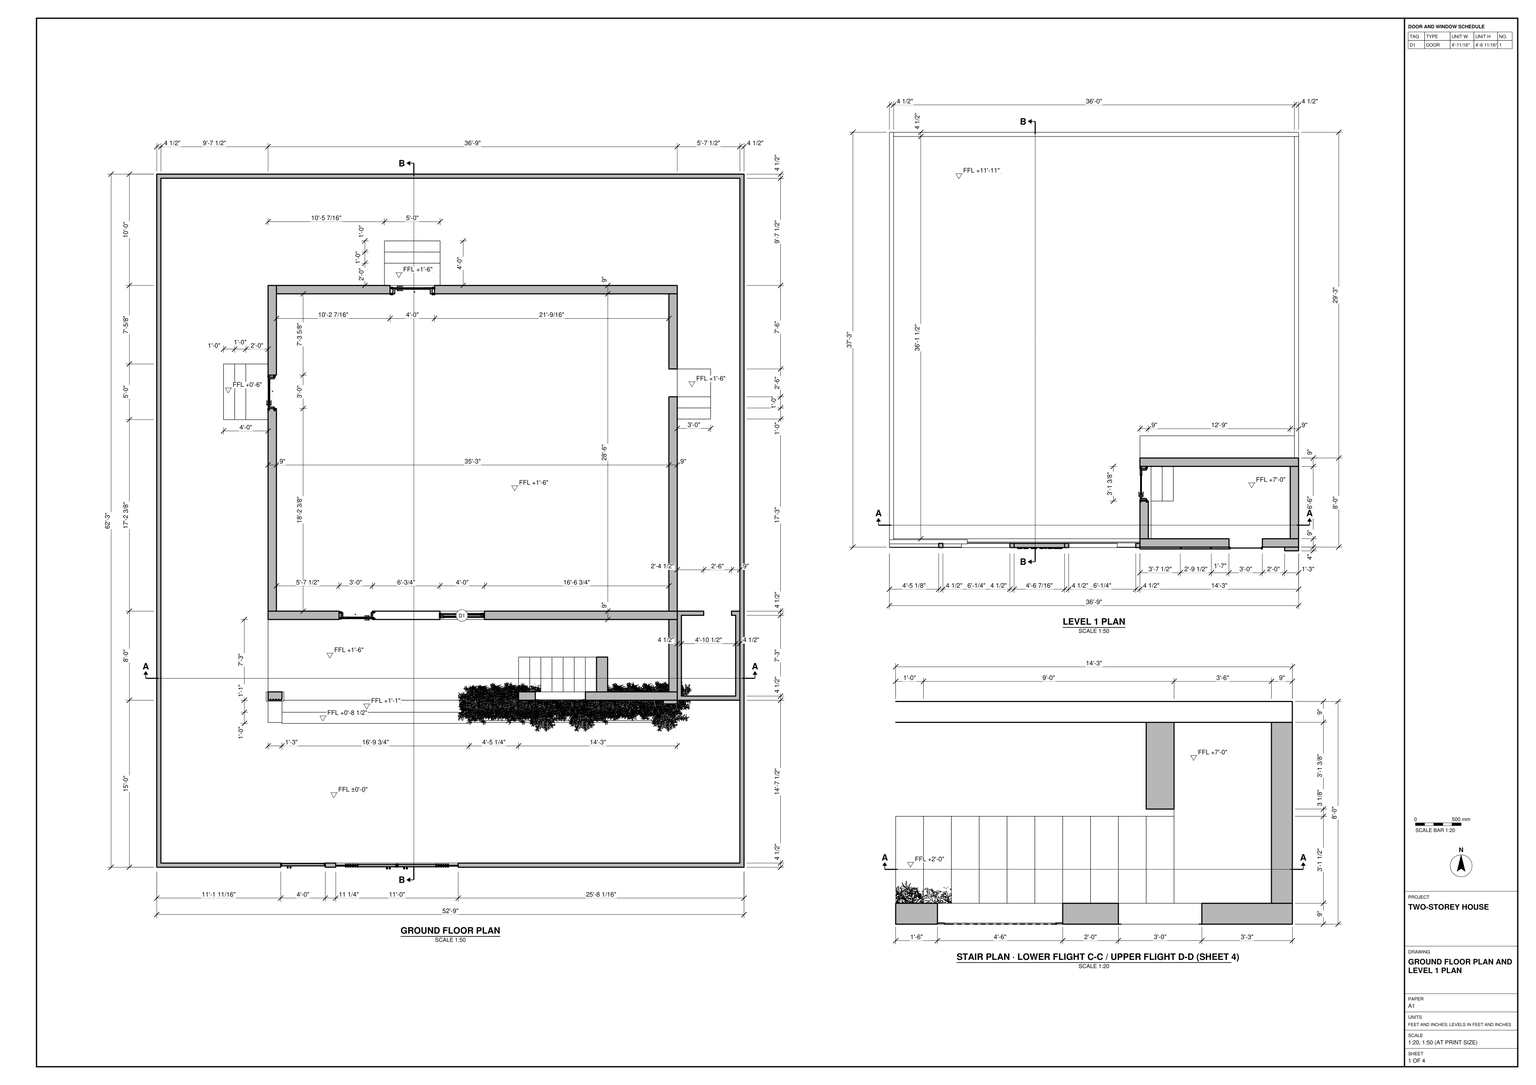
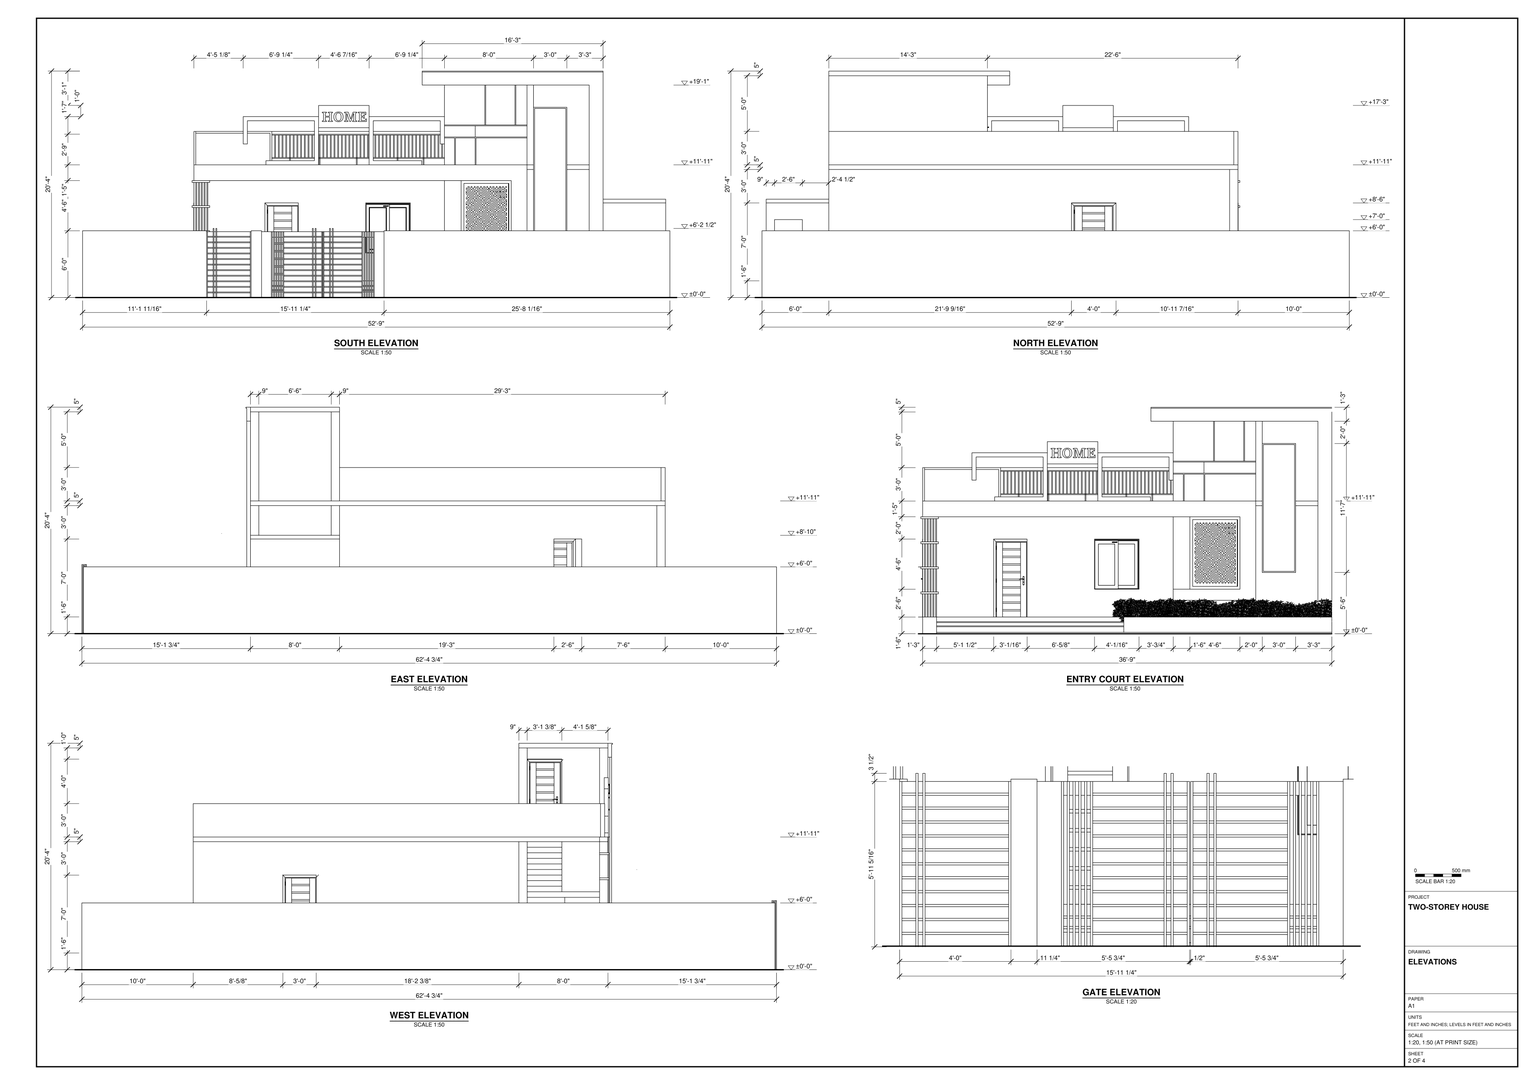
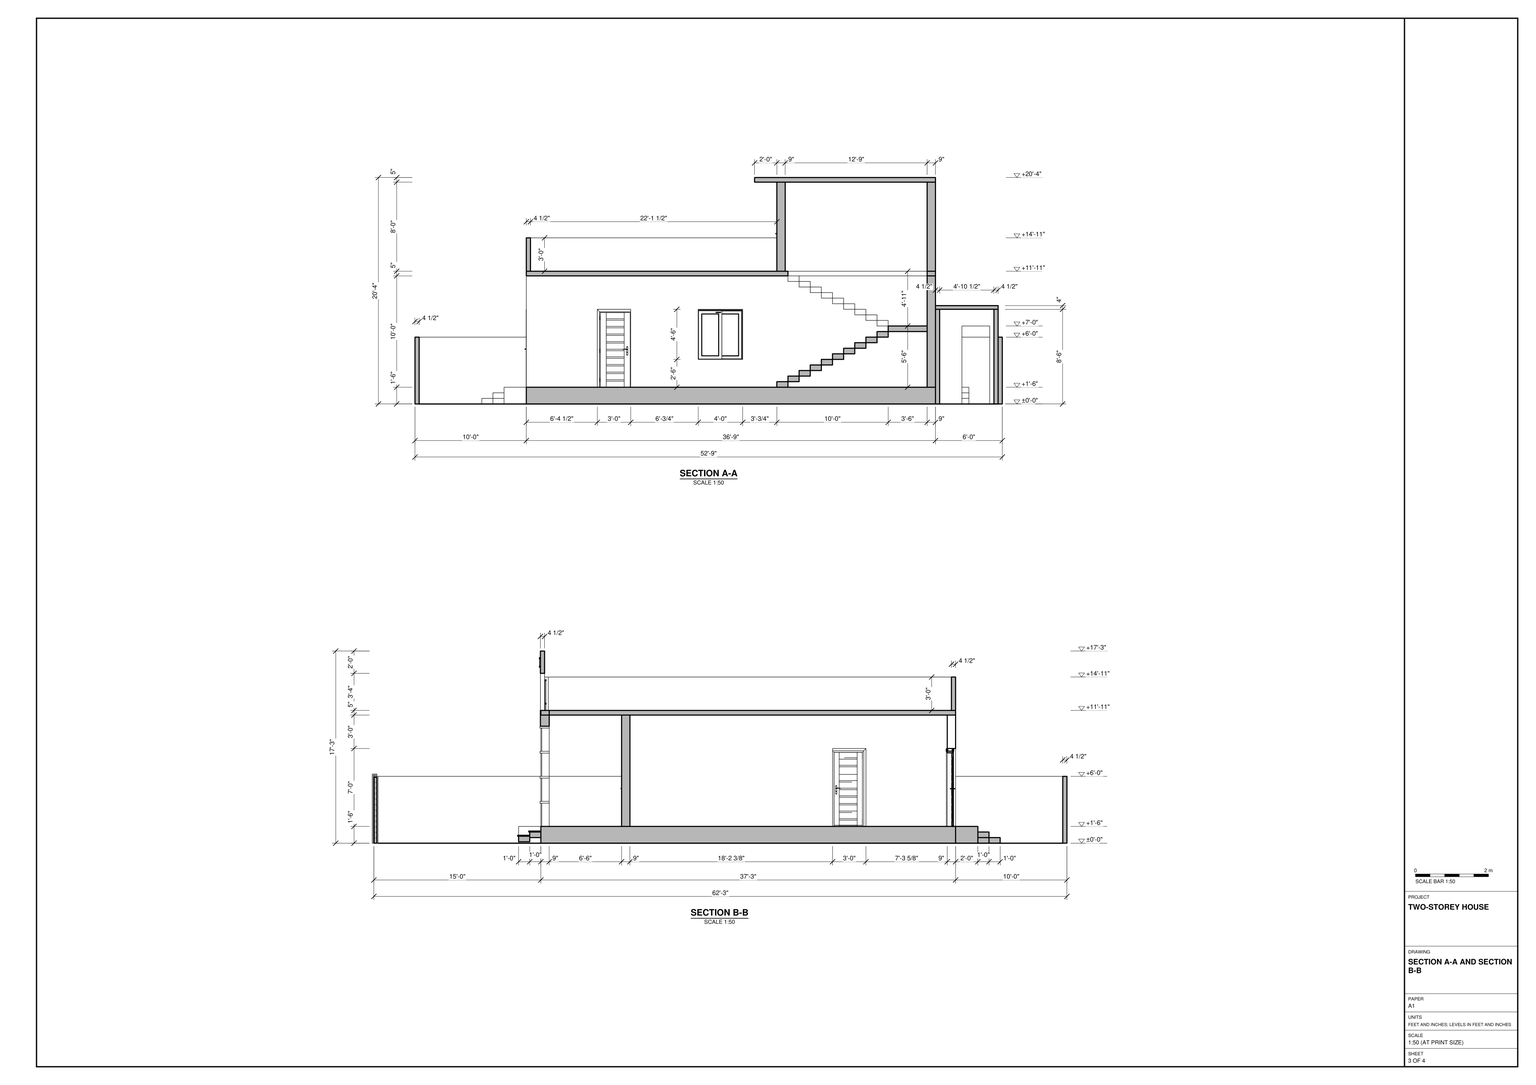
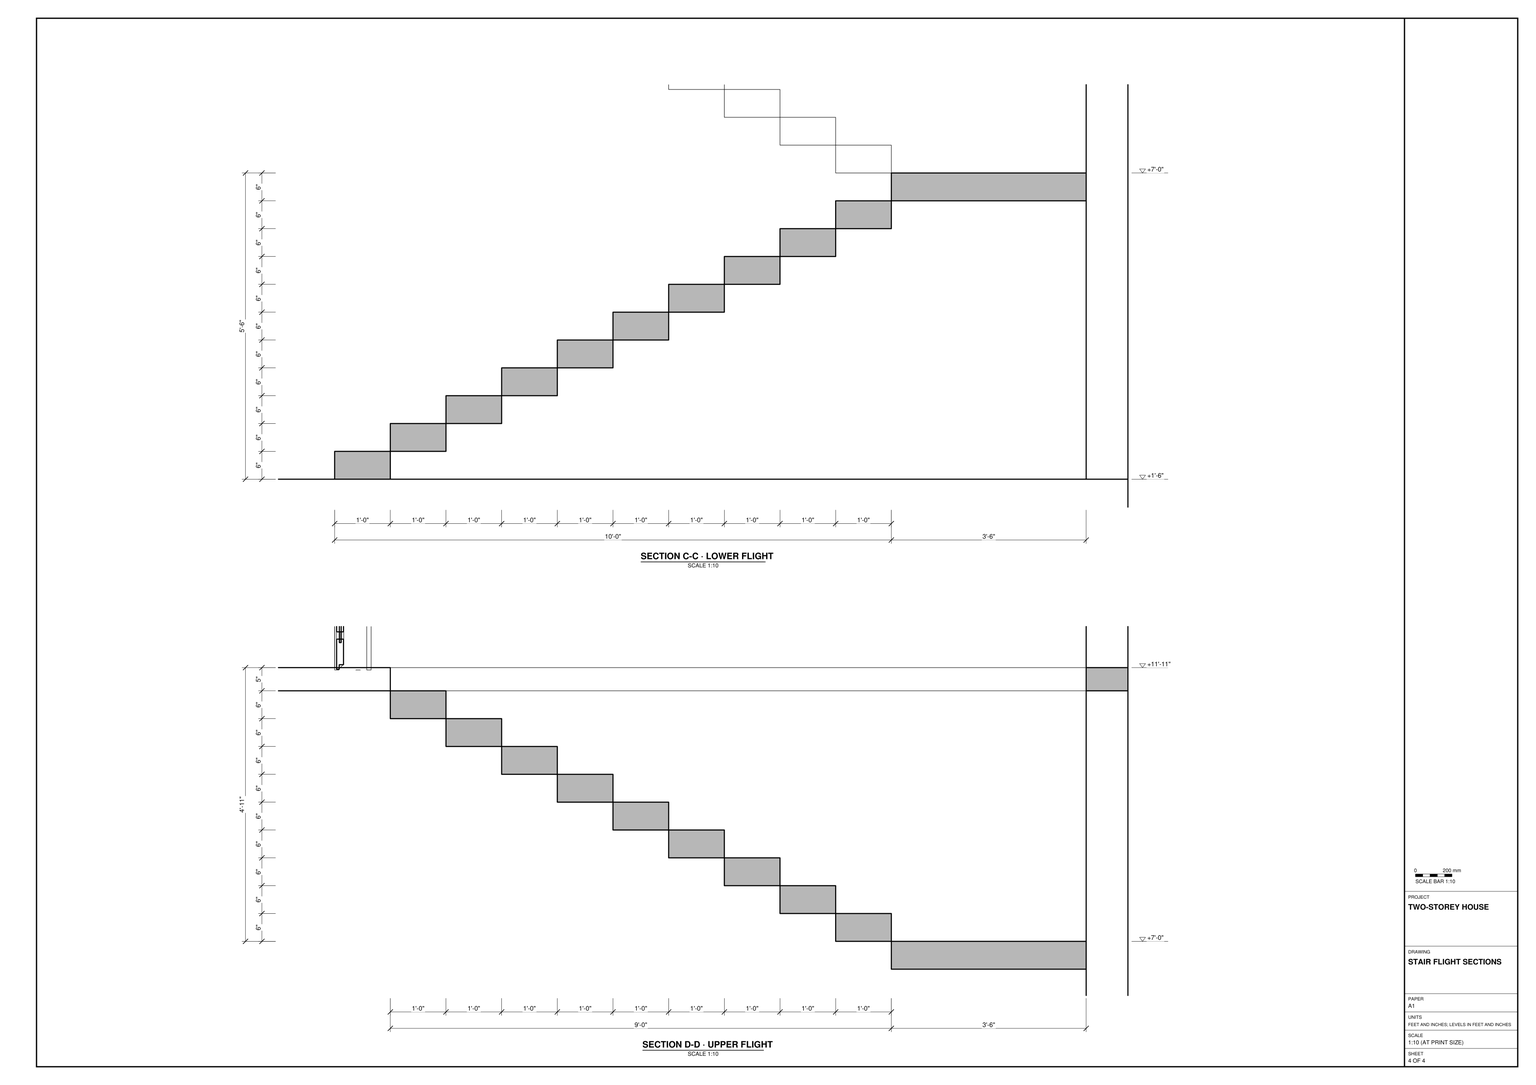
Build the house and its enclosed site in SketchUp from task_files/diagram_01.pdf. Work in feet and inches. Including the site walls, the model measures 52'-9" east to west, 62'-4 3/4" north to south and 20'-4 5/16" high. Use ±0'-0" as the ground datum and +11'-11" as the upper level.

Set the house back from the south gate to leave the entry court shown in plan. Model the raised floor slab, entrance steps and landings, keeping the main floor at +1'-6" above the court. Follow the wall faces and openings on the plans, distinguishing the 9" main walls from the 4 1/2" perimeter walls. Fit the doors and window units shown in elevation. On the court side, include the screened panel, the planted strip and the barred pedestrian and vehicle gates.

Build the return stair at the southeast corner with two flights and an intermediate landing. Align the upper flight with the roof terrace and model the stair enclosure with its projecting flat roof. Use the sections to set the slabs and parapets, and the entry court elevation to lay out the front railing and its central panel. Decor and loose items, including the shrubs, may be any suitable library components.

Keep shell elements such as walls, slabs and roofs, and each furniture or joinery piece shown, in separate groups or components. Use components for repeated parts. Save one SketchUp model as output_files/two_storey_house_with_a_gated_court_and_roof_terrace.skp.

# SketchUp Ruby script. Lengths in inches.
U = 1.inch
M = Sketchup.active_model
def pt(a) = Geom::Point3d.new(a.map { |v| v * U })
def face(e, loops, mat)
  f = e.add_face(loops[0].map { |a| pt(a) })
  loops[1..].each { |l| e.add_face(l.map { |a| pt(a) }).erase! }
  f.material = f.back_material = mat if mat
  f
end
# faces: each face lists its corners as indices into pts; further lists are holes
def faces(e, pts, list, mat = nil) = list.each { |f| face(e, (f[0].is_a?(Array) ? f : [f]).map { |l| l.map { |i| pts[i] } }, mat) }
# xy, xz, yz: faces in a plane at the given z, y or x. An outline is a flat list of corners, or four numbers for a rectangle; further outlines are holes
def ring(l) = l.size == 4 ? [[l[0], l[1]], [l[2], l[1]], [l[2], l[3]], [l[0], l[3]]] : l.each_slice(2).to_a
def flat(e, list, mat, &to3) = list.each { |f| face(e, (f[0].is_a?(Array) ? f : [f]).map { |l| ring(l).map { |u, v| to3.(u, v) } }, mat) }
def xy(e, z, list, mat = nil) = flat(e, list, mat) { |x, y| [x, y, z] }
def xz(e, y, list, mat = nil) = flat(e, list, mat) { |x, z| [x, y, z] }
def yz(e, x, list, mat = nil) = flat(e, list, mat) { |y, z| [x, y, z] }
def lines(e, pts, list) = list.each { |a, b| e.add_line(pt(pts[a]), pt(pts[b])) }
# prism: a flat outline (further loops are holes) pulled along v
def prism(e, loops, v, mat = nil)
  f = face(e, loops, mat); d = Geom::Vector3d.new(v.map { |x| x * U })
  f.pushpull(f.normal.samedirection?(d) ? d.length : -d.length)
end
def box(e, o, s, mat = nil) = prism(e, [[o, [o[0] + s[0], o[1], o[2]], [o[0] + s[0], o[1] + s[1], o[2]], [o[0], o[1] + s[1], o[2]]]], [0, 0, s[2]], mat)
def at(x, y, z, deg = 0) = Geom::Transformation.translation(pt([x, y, z])) * Geom::Transformation.rotation(ORIGIN, Z_AXIS, deg.degrees)
def axes(o, x, y, z) = Geom::Transformation.new([*x, 0, *y, 0, *z, 0, *pt(o).to_a, 1])
def part(name) = M.definitions.add(name)
# library, detail: a bought-in or finely detailed component or shape, given as its bounding box
def library(name, o, s) = part(name).tap { |d| box(d.entities, o, s) }
def detail(e, o, s) = box(e.add_group.entities, o, s)
def put(e, d, t, mat = nil) = e.add_instance(d, t).tap { |i| i.material = mat if mat }
def group(e, t, mat = nil) = e.add_group.tap { |g| g.transformation = t; g.material = mat if mat }.entities
root = M.entities
M.materials.add("B06_Amber_Rust1").color = [177, 136, 101]
M.materials.add("Glass_Basic_01").color = [161, 173, 186]
M.materials["Glass_Basic_01"].alpha = 0.25
M.materials.add("L04_Berry_Fizz1").color = [175, 199, 193]
M.materials.add("L08_Velvet_Rose1").color = [231, 225, 220]
M.materials.add("M00_Soft_Cloud").color = [255, 255, 255]
M.materials.add("M03_Pewter_Shine").color = [168, 168, 168]
M.materials.add("M05_Graphite_Haze").color = [114, 114, 114]
M.materials.add("M06_Steel_Smoke").color = [86, 86, 86]
M.materials.add("M07_Charcoal_Gleam").color = [58, 58, 58]
M.materials.add("[0131_Silver]").color = [192, 192, 192]
c1 = library("Group6\#1",[-22.44,-5.97,0],[42.52,9.29,84.25])
c2 = library("AS-120-mm",[0,0,0],[48.66,4.72,54.66])
c3 = library("00_SHRUBS",[-11.28,-20.125,-2.03],[165.95,98.02,60.68])
c4 = library("HOME",[0.71,0,0],[47.66,10.57,1])
c5 = part("Group\#8")
box(c5.entities,[0,0,0],[12,37.5,6])
c6 = part("Group82\#1")
p = [[-1.1875,137.8125,0],[-1.1875,1.1875,0],[-34.8125,1.1875,0],[-34.8125,137.8125,0]]
lines(c6.entities,p,[[0,1],[1,2],[2,3],[3,0]])
c7 = part("Group83\#1")
xy(c7.entities,1,[[-34.8125,1.1875,-1.1875,137.8125]])
c8 = part("Group81\#1")
prism(c8.entities,[[[-36,139,0],[0,139,0],[0,0,0],[-36,0,0]],[[-34.8125,1.1875,0],[-1.1875,1.1875,0],[-1.1875,137.8125,0],[-34.8125,137.8125,0]]],[0,0,2])
put(c8.entities,c6,at(0,0,0))
put(c8.entities,c7,at(0,0,0),"Glass_Basic_01")
c9 = library("Group\#16",[0,0,0],[54,1.5,78])
c10 = part("Group\#19")
prism(c10.entities,[[[4.5,4.5,22.51],[0,4.5,22.51],[0,4.5,52],[81.24,4.5,52],[81.24,4.5,0],[24.49,4.5,0],[24.49,4.5,4.5],[76.74,4.5,4.5],[76.74,4.5,47.5],[4.5,4.5,47.5]]],[0,-4.5,0])
c11 = part("Group\#20")
box(c11.entities,[0,0,0],[186.02,1,1])
c12 = part("Group\#27")
box(c12.entities,[0,0,0],[1,1,24.15])
c13 = part("Group\#29")
box(c13.entities,[0,0,0],[201.78,12,6])
c14 = part("Group\#32")
box(c14.entities,[0,0,0],[201.78,13,1])
c15 = part("Group\#39")
prism(c15.entities,[[[0,0,0],[0,10,0],[2,10,0],[2,1,0],[17,1,0],[17,10,0],[19,10,0],[19,0,0]]],[0,0,2])
c16 = part("Vertical gate bar")
box(c16.entities,[0,0,0],[1,1,71])
c17 = part("Gate stile")
box(c17.entities,[0,0,0],[1,3,71],"[0131_Silver]")
c18 = part("Driveway gate leaf")
xy(c18.entities,0,[[24,0,64.75,3]])
xy(c18.entities,0,[[0,1,24,2]],"[0131_Silver]")
xy(c18.entities,5,[[24,0,64.75,0.25],[24,2.75,64.75,3]],"[0131_Silver]")
xy(c18.entities,6,[[24,0,64.75,0.25],[10.5,1,24,2],[24,2.75,64.75,3]],"[0131_Silver]")
xy(c18.entities,11,[[24,0,64.75,0.25],[24,2.75,64.75,3]],"[0131_Silver]")
xy(c18.entities,12,[[24,0,64.75,0.25],[24,2.75,64.75,3]],"[0131_Silver]")
xy(c18.entities,17,[[24,0,64.75,0.25],[24,2.75,64.75,3]],"[0131_Silver]")
xy(c18.entities,18,[[24,0,64.75,0.25],[24,2.75,64.75,3]],"[0131_Silver]")
xy(c18.entities,23,[[24,0,64.75,0.25],[24,2.75,64.75,3]],"[0131_Silver]")
xy(c18.entities,24,[[24,0,64.75,0.25],[24,2.75,64.75,3]],"[0131_Silver]")
xy(c18.entities,29,[[24,0,64.75,0.25],[24,2.75,64.75,3]],"[0131_Silver]")
xy(c18.entities,30,[[24,0,64.75,0.25],[24,2.75,64.75,3]],"[0131_Silver]")
xy(c18.entities,35,[[24,0,64.75,0.25],[24,2.75,64.75,3]],"[0131_Silver]")
xy(c18.entities,36,[[24,0,64.75,0.25],[24,2.75,64.75,3]],"[0131_Silver]")
xy(c18.entities,41,[[24,0,64.75,0.25],[24,2.75,64.75,3]],"[0131_Silver]")
xy(c18.entities,42,[[24,0,64.75,0.25],[24,2.75,64.75,3]],"[0131_Silver]")
xy(c18.entities,47,[[24,0,64.75,0.25],[24,2.75,64.75,3]],"[0131_Silver]")
xy(c18.entities,48,[[24,0,64.75,0.25],[24,2.75,64.75,3]],"[0131_Silver]")
xy(c18.entities,53,[[24,0,64.75,0.25],[24,2.75,64.75,3]],"[0131_Silver]")
xy(c18.entities,54,[[24,0,64.75,0.25],[24,2.75,64.75,3]],"[0131_Silver]")
xy(c18.entities,59,[[24,0,64.75,0.25],[24,2.75,64.75,3]],"[0131_Silver]")
xy(c18.entities,60,[[24,0,64.75,0.25],[24,2.75,64.75,3]],"[0131_Silver]")
xy(c18.entities,65,[[10.5,1,24,2]])
xy(c18.entities,65,[[24,0,64.75,0.25],[24,2.75,64.75,3]],"[0131_Silver]")
xy(c18.entities,66,[[24,0,64.75,0.25],[24,2.75,64.75,3]],"[0131_Silver]")
xy(c18.entities,71,[[24,0,64.75,3]])
xy(c18.entities,71,[[0,1,24,2]],"[0131_Silver]")
xz(c18.entities,0,[[24,0,64.75,5],[24,6,64.75,11],[24,12,64.75,17],[24,18,64.75,23],[24,24,64.75,29],
  [24,30,64.75,35],[24,36,64.75,41],[24,42,64.75,47],[24,48,64.75,53],[24,54,64.75,59],
  [24,60,64.75,65],[24,66,64.75,71]])
xz(c18.entities,0.25,[[24,5,64.75,6],[24,11,64.75,12],[24,17,64.75,18],[24,23,64.75,24],[24,29,64.75,30],
  [24,35,64.75,36],[24,41,64.75,42],[24,47,64.75,48],[24,53,64.75,54],[24,59,64.75,60],
  [24,65,64.75,66]],"[0131_Silver]")
xz(c18.entities,1,[[0,0,24,0,24,6,10.5,6,10.5,65,24,65,24,71,0,71]],"[0131_Silver]")
xz(c18.entities,2,[[0,0,0,71,24,71,24,65,10.5,65,10.5,6,24,6,24,0]],"[0131_Silver]")
xz(c18.entities,2.75,[[24,5,64.75,6],[24,11,64.75,12],[24,17,64.75,18],[24,23,64.75,24],[24,29,64.75,30],
  [24,35,64.75,36],[24,41,64.75,42],[24,47,64.75,48],[24,53,64.75,54],[24,59,64.75,60],
  [24,65,64.75,66]],"[0131_Silver]")
xz(c18.entities,3,[[24,0,64.75,5],[24,6,64.75,11],[24,12,64.75,17],[24,18,64.75,23],[24,24,64.75,29],
  [24,30,64.75,35],[24,36,64.75,41],[24,42,64.75,47],[24,48,64.75,53],[24,54,64.75,59],
  [24,60,64.75,65],[24,66,64.75,71]])
yz(c18.entities,0,[[1,0,2,71]],"[0131_Silver]")
yz(c18.entities,10.5,[[1,6,2,65]],"[0131_Silver]")
yz(c18.entities,24,[[0,0,1,5],[1,0,2,6],[2,0,2,6,2.75,6,2.75,5,3,5,3,0],[0.25,5,0.25,6,0,6,0,11,0.25,11,0.25,12,0,12,0,17,0.25,17,0.25,18,0,18,0,23,0.25,23,0.25,24,0,24,0,29,0.25,29,0.25,30,0,30,0,35,0.25,35,0.25,36,0,36,0,41,0.25,41,0.25,42,0,42,0,47,0.25,47,0.25,48,0,48,0,53,0.25,53,0.25,54,0,54,0,59,0.25,59,0.25,60,0,60,0,65,3,65,3,60,2.75,60,2.75,59,3,59,3,54,2.75,54,2.75,53,3,53,3,48,2.75,48,2.75,47,3,47,3,42,2.75,42,2.75,41,3,41,3,36,2.75,36,2.75,35,3,35,3,30,2.75,30,2.75,29,3,29,3,24,2.75,24,2.75,23,3,23,3,18,2.75,18,2.75,17,3,17,3,12,2.75,12,2.75,11,3,11,3,6,1,6,1,5],[0.25,65,0.25,66,0,66,0,71,1,71,1,65],
  [1,65,2,71],[2,65,2,71,3,71,3,66,2.75,66,2.75,65]])
yz(c18.entities,64.75,[[0,0,3,0,3,5,2.75,5,2.75,6,3,6,3,11,2.75,11,2.75,12,3,12,3,17,2.75,17,2.75,18,3,18,3,23,2.75,23,2.75,24,3,24,3,29,2.75,29,2.75,30,3,30,3,35,2.75,35,2.75,36,3,36,3,41,2.75,41,2.75,42,3,42,3,47,2.75,47,2.75,48,3,48,3,53,2.75,53,2.75,54,3,54,3,59,2.75,59,2.75,60,3,60,3,65,2.75,65,2.75,66,3,66,3,71,0,71,0,66,0.25,66,0.25,65,0,65,0,60,0.25,60,0.25,59,0,59,0,54,0.25,54,0.25,53,0,53,0,48,0.25,48,0.25,47,0,47,0,42,0.25,42,0.25,41,0,41,0,36,0.25,36,0.25,35,0,35,0,30,0.25,30,0.25,29,0,29,0,24,0.25,24,0.25,23,0,23,0,18,0.25,18,0.25,17,0,17,0,12,0.25,12,0.25,11,0,11,0,6,0.25,6,0.25,5,0,5]])
put(c18.entities,c16,at(10.5,0,0),"[0131_Silver]")
put(c18.entities,c16,at(10.5,2,0),"[0131_Silver]")
put(c18.entities,c16,at(13,2,0),"[0131_Silver]")
put(c18.entities,c16,at(13,0,0),"[0131_Silver]")
put(c18.entities,c16,at(15.5,0,0),"[0131_Silver]")
put(c18.entities,c16,at(18,0,0),"[0131_Silver]")
put(c18.entities,c16,at(20.5,0,0),"[0131_Silver]")
put(c18.entities,c17,at(64.75,0,0),"[0131_Silver]")
put(c18.entities,c16,at(23,0,0),"[0131_Silver]")
put(c18.entities,c16,at(15.5,2,0),"[0131_Silver]")
put(c18.entities,c16,at(18,2,0),"[0131_Silver]")
put(c18.entities,c16,at(20.5,2,0),"[0131_Silver]")
put(c18.entities,c16,at(23,2,0),"[0131_Silver]")
c19 = part("Gate pull handle")
prism(c19.entities,[[[0,1,0],[0,0,0],[0,0,2.5],[0,-2,2.5],[0,-2,-70.3125],[0,-1,-70.3125],[0,-1,-71.3125],[0,-3,-71.3125],[0,-3,3.5],[0,1,3.5]]],[1,0,0])
c20 = part("Double driveway gate")
put(c20.entities,c18,at(0,2,0.3125))
put(c20.entities,c18,axes([132,2,0.3125],[-1,0,0],[0,1,0],[0,0,1]))
put(c20.entities,c19,at(57.75,3,71.3125),"[0131_Silver]")
put(c20.entities,c19,at(54.75,3,71.3125),"[0131_Silver]")
put(c20.entities,c19,at(73.25,3,71.3125),"[0131_Silver]")
put(c20.entities,c19,at(76.25,3,71.3125),"[0131_Silver]")
c21 = part("Pedestrian gate")
xy(c21.entities,0.3125,[[1,2,47,5]])
xy(c21.entities,5.3125,[[1,2,47,2.25],[1,4.75,47,5]],"[0131_Silver]")
xy(c21.entities,6.3125,[[1,2,47,2.25],[1,4.75,47,5]],"[0131_Silver]")
xy(c21.entities,11.3125,[[1,2,47,2.25],[1,4.75,47,5]],"[0131_Silver]")
xy(c21.entities,12.3125,[[1,2,47,2.25],[1,4.75,47,5]],"[0131_Silver]")
xy(c21.entities,17.3125,[[1,2,47,2.25],[1,4.75,47,5]],"[0131_Silver]")
xy(c21.entities,18.3125,[[1,2,47,2.25],[1,4.75,47,5]],"[0131_Silver]")
xy(c21.entities,23.3125,[[1,2,47,2.25],[1,4.75,47,5]],"[0131_Silver]")
xy(c21.entities,24.3125,[[1,2,47,2.25],[1,4.75,47,5]],"[0131_Silver]")
xy(c21.entities,29.3125,[[1,2,47,2.25],[1,4.75,47,5]],"[0131_Silver]")
xy(c21.entities,30.3125,[[1,2,47,2.25],[1,4.75,47,5]],"[0131_Silver]")
xy(c21.entities,35.3125,[[1,2,47,2.25],[1,4.75,47,5]],"[0131_Silver]")
xy(c21.entities,36.3125,[[1,2,47,2.25],[1,4.75,47,5]],"[0131_Silver]")
xy(c21.entities,41.3125,[[1,2,47,2.25],[1,4.75,47,5]],"[0131_Silver]")
xy(c21.entities,42.3125,[[1,2,47,2.25],[1,4.75,47,5]],"[0131_Silver]")
xy(c21.entities,47.3125,[[1,2,47,2.25],[1,4.75,47,5]],"[0131_Silver]")
xy(c21.entities,48.3125,[[1,2,47,2.25],[1,4.75,47,5]],"[0131_Silver]")
xy(c21.entities,53.3125,[[1,2,47,2.25],[1,4.75,47,5]],"[0131_Silver]")
xy(c21.entities,54.3125,[[1,2,47,2.25],[1,4.75,47,5]],"[0131_Silver]")
xy(c21.entities,59.3125,[[1,2,47,2.25],[1,4.75,47,5]],"[0131_Silver]")
xy(c21.entities,60.3125,[[1,2,47,2.25],[1,4.75,47,5]],"[0131_Silver]")
xy(c21.entities,65.3125,[[1,2,47,2.25],[1,4.75,47,5]],"[0131_Silver]")
xy(c21.entities,66.3125,[[1,2,47,2.25],[1,4.75,47,5]],"[0131_Silver]")
xy(c21.entities,71.3125,[[1,2,47,5]])
xz(c21.entities,2,[[1,0.3125,47,5.3125],[1,6.3125,47,11.3125],[1,12.3125,47,17.3125],[1,18.3125,47,23.3125],[1,24.3125,47,29.3125],
  [1,30.3125,47,35.3125],[1,36.3125,47,41.3125],[1,42.3125,47,47.3125],[1,48.3125,47,53.3125],[1,54.3125,47,59.3125],
  [1,60.3125,47,65.3125],[1,66.3125,47,71.3125]])
xz(c21.entities,2.25,[[1,5.3125,47,6.3125],[1,11.3125,47,12.3125],[1,17.3125,47,18.3125],[1,23.3125,47,24.3125],[1,29.3125,47,30.3125],
  [1,35.3125,47,36.3125],[1,41.3125,47,42.3125],[1,47.3125,47,48.3125],[1,53.3125,47,54.3125],[1,59.3125,47,60.3125],
  [1,65.3125,47,66.3125]],"[0131_Silver]")
xz(c21.entities,4.75,[[1,5.3125,47,6.3125],[1,11.3125,47,12.3125],[1,17.3125,47,18.3125],[1,23.3125,47,24.3125],[1,29.3125,47,30.3125],
  [1,35.3125,47,36.3125],[1,41.3125,47,42.3125],[1,47.3125,47,48.3125],[1,53.3125,47,54.3125],[1,59.3125,47,60.3125],
  [1,65.3125,47,66.3125]],"[0131_Silver]")
xz(c21.entities,5,[[1,0.3125,47,5.3125],[1,6.3125,47,11.3125],[1,12.3125,47,17.3125],[1,18.3125,47,23.3125],[1,24.3125,47,29.3125],
  [1,30.3125,47,35.3125],[1,36.3125,47,41.3125],[1,42.3125,47,47.3125],[1,48.3125,47,53.3125],[1,54.3125,47,59.3125],
  [1,60.3125,47,65.3125],[1,66.3125,47,71.3125]])
yz(c21.entities,1,[[2,0.3125,3,5.3125],[3,0.3125,4,6.3125],[4,0.3125,4,6.3125,4.75,6.3125,4.75,5.3125,5,5.3125,5,0.3125],[2.25,5.3125,2.25,6.3125,2,6.3125,2,11.3125,2.25,11.3125,2.25,12.3125,2,12.3125,2,17.3125,2.25,17.3125,2.25,18.3125,2,18.3125,2,23.3125,2.25,23.3125,2.25,24.3125,2,24.3125,2,29.3125,2.25,29.3125,2.25,30.3125,2,30.3125,2,35.3125,2.25,35.3125,2.25,36.3125,2,36.3125,2,41.3125,2.25,41.3125,2.25,42.3125,2,42.3125,2,47.3125,2.25,47.3125,2.25,48.3125,2,48.3125,2,53.3125,2.25,53.3125,2.25,54.3125,2,54.3125,2,59.3125,2.25,59.3125,2.25,60.3125,2,60.3125,2,65.3125,5,65.3125,5,60.3125,4.75,60.3125,4.75,59.3125,5,59.3125,5,54.3125,4.75,54.3125,4.75,53.3125,5,53.3125,5,48.3125,4.75,48.3125,4.75,47.3125,5,47.3125,5,42.3125,4.75,42.3125,4.75,41.3125,5,41.3125,5,36.3125,4.75,36.3125,4.75,35.3125,5,35.3125,5,30.3125,4.75,30.3125,4.75,29.3125,5,29.3125,5,24.3125,4.75,24.3125,4.75,23.3125,5,23.3125,5,18.3125,4.75,18.3125,4.75,17.3125,5,17.3125,5,12.3125,4.75,12.3125,4.75,11.3125,5,11.3125,5,6.3125,3,6.3125,3,5.3125],[2.25,65.3125,2.25,66.3125,2,66.3125,2,71.3125,3,71.3125,3,65.3125],
  [3,65.3125,4,71.3125],[4,65.3125,4,71.3125,5,71.3125,5,66.3125,4.75,66.3125,4.75,65.3125]])
yz(c21.entities,47,[[2,0.3125,5,0.3125,5,5.3125,4.75,5.3125,4.75,6.3125,5,6.3125,5,11.3125,4.75,11.3125,4.75,12.3125,5,12.3125,5,17.3125,4.75,17.3125,4.75,18.3125,5,18.3125,5,23.3125,4.75,23.3125,4.75,24.3125,5,24.3125,5,29.3125,4.75,29.3125,4.75,30.3125,5,30.3125,5,35.3125,4.75,35.3125,4.75,36.3125,5,36.3125,5,41.3125,4.75,41.3125,4.75,42.3125,5,42.3125,5,47.3125,4.75,47.3125,4.75,48.3125,5,48.3125,5,53.3125,4.75,53.3125,4.75,54.3125,5,54.3125,5,59.3125,4.75,59.3125,4.75,60.3125,5,60.3125,5,65.3125,4.75,65.3125,4.75,66.3125,5,66.3125,5,71.3125,2,71.3125,2,66.3125,2.25,66.3125,2.25,65.3125,2,65.3125,2,60.3125,2.25,60.3125,2.25,59.3125,2,59.3125,2,54.3125,2.25,54.3125,2.25,53.3125,2,53.3125,2,48.3125,2.25,48.3125,2.25,47.3125,2,47.3125,2,42.3125,2.25,42.3125,2.25,41.3125,2,41.3125,2,36.3125,2.25,36.3125,2.25,35.3125,2,35.3125,2,30.3125,2.25,30.3125,2.25,29.3125,2,29.3125,2,24.3125,2.25,24.3125,2.25,23.3125,2,23.3125,2,18.3125,2.25,18.3125,2.25,17.3125,2,17.3125,2,12.3125,2.25,12.3125,2.25,11.3125,2,11.3125,2,6.3125,2.25,6.3125,2.25,5.3125,2,5.3125]])
p = [[0,2,71.3125],[1,2,71.3125]]
lines(c21.entities,p,[[0,1]])
put(c21.entities,c17,at(0,2,0.3125),"[0131_Silver]")
put(c21.entities,c17,at(47,2,0.3125),"[0131_Silver]")
put(c21.entities,c19,at(40,3,71.3125),"[0131_Silver]")
put(c21.entities,c19,at(37,3,71.3125),"[0131_Silver]")
c22 = part("Group\#35")
box(c22.entities,[0,0,0],[12,60,6])
c23 = part("Group\#48")
g1 = group(c23.entities,at(12,0,0.02))
box(g1,[0,0,0],[12,60,6])
g2 = group(c23.entities,at(24,12,1.5))
box(g2,[0,-12,-1.5],[24,60,18.02])
put(c23.entities,c22,at(0,0,0.02))
put(c23.entities,c22,at(12,0,6.02))
c24 = part("Group\#51")
box(c24.entities,[0,0,0],[36,12,6])
box(root,[561,181.74,83.98],[67.5,96,4])
p = [[387.11,150.61,89.94],[387.11,150.57,89.94],[379.61,150.61,89.94],[379.61,150.57,89.94]]
lines(root,p,[[0,1],[2,3]])
put(root,c1,axes([214.74,273.87,-0.16],[-0.91,0,0],[0,1,0],[0,0,0.99888]))
put(root,c2,at(304.59,270.73,29.34))
put(root,c3,axes([455.8125,147.79,-16.46],[0.81,0,0],[0,0.81,0],[0,0,0.81]))
put(root,c3,axes([366.48,147.79,-16.46],[0.81,0,0],[0,0.81,0],[0,0,0.81]))
put(root,c3,axes([324.1,147.79,-16.46],[0.81,0,0],[0,0.81,0],[0,0,0.81]))
put(root,c4,axes([257.57,181.24,171.43],[1,0,0],[0,0,1],[0,-1,0]))
put(root,c1,axes([124.36,514.04,0.12],[0,0.91,0],[1,0,0],[0,0,0.99888]))
put(root,c1,axes([277.05,622.07,-0.32],[1.14059,0,0],[0,-1,0],[0,0,0.99888]))
put(root,c1,axes([394.55,250.54,124.49],[0,0.91,0],[1,0,0],[0,0,0.99888]))
g3 = group(root,at(120,268.74,0))
prism(g3,[[[0,0,0],[76.5,0,0],[76.5,0,84],[112.5,0,84],[112.5,0,0],[441,0,0],[441,0,120],[0,0,120]],[[185.25,0,30],[185.25,0,84],[233.25,0,84],[233.25,0,30]]],[0,9,0])
g4 = group(root,at(120,277.74,0))
prism(g4,[[[9,254.39,0],[9,351,0],[9,351,120],[9,0,120],[9,0,0],[9,218.39,0],[9,218.39,84],[9,254.39,84]]],[-9,0,0])
g5 = group(root,at(129,619.74,0))
prism(g5,[[[432,9,0],[170.45,9,0],[170.45,9,84],[122.45,9,84],[122.45,9,0],[0,9,0],[0,9,120],[432,9,120]]],[0,-9,0])
g6 = group(root,at(552,277.74,0))
prism(g6,[[[0,342,0],[0,261,0],[0,261,84],[0,231,84],[0,231,0],[0,0,0],[0,0,120],[0,342,120]]],[9,0,0])
g7 = group(root,at(552,190.74,0))
box(g7,[0,0,0],[9,78,120])
g8 = group(root,at(336.78,181.74,0))
xy(g8,0,[[53.22,0,224.22,9]])
xy(g8,30,[[71.22,0,125.22,9]])
xy(g8,48,[[149.22,0,185.22,9]])
xy(g8,108,[[71.22,0,125.22,9]])
xy(g8,120,[[53.22,0,149.22,9],[185.22,0,224.22,9]])
xz(g8,0,[[142.07,0,224.22,0,224.22,120,185.22,120,185.22,48,149.22,48,149.22,120,142.07,120]],"L04_Berry_Fizz1")
xz(g8,0,[[53.22,0,142.07,0,142.07,120,53.22,120,53.22,108,125.22,108,125.22,30,53.22,30]],"L08_Velvet_Rose1")
xz(g8,0,[[53.22,30,71.22,108]],"M00_Soft_Cloud")
xz(g8,9,[[[53.22,0,53.22,120,149.22,120,149.22,48,185.22,48,185.22,120,224.22,120,224.22,0],[71.22,30,125.22,108]]])
yz(g8,53.22,[[0,0,9,120]])
yz(g8,71.22,[[0,30,9,108]])
yz(g8,125.22,[[0,30,9,108]])
yz(g8,149.22,[[0,48,9,120]])
yz(g8,185.22,[[0,48,9,120]])
yz(g8,224.22,[[0,0,9,120]])
g9 = group(root,at(390,268.74,0))
put(g9,c5,axes([12,-40.5,6],[1,0,0],[0,-1,0],[0,0,1]))
put(g9,c5,axes([0,-40.5,0],[1,0,0],[0,-1,0],[0,0,1]))
put(g9,c5,axes([84,0,78],[1,0,0],[0,-0.99686,0],[0,0,1]))
put(g9,c5,axes([48,0,96],[1,0,0],[0,-0.99686,0],[0,0,1]))
put(g9,c5,axes([96,0,72],[1,0,0],[0,-0.99686,0],[0,0,1]))
put(g9,c5,axes([72,0,84],[1,0,0],[0,-0.99686,0],[0,0,1]))
put(g9,c5,axes([60,0,90],[1,0,0],[0,-0.99686,0],[0,0,1]))
put(g9,c5,axes([24,0,108],[1,0,0],[0,-0.99686,0],[0,0,1]))
put(g9,c5,axes([12,0,114],[1,0,0],[0,-0.99686,0],[0,0,1]))
put(g9,c5,axes([36,0,102],[1,0,0],[0,-0.99686,0],[0,0,1]))
put(g9,c5,axes([108,0,66],[1,0,0],[0,-0.99686,0],[0,0,1]))
put(g9,c5,axes([96,-40.5,48],[1,0,0],[0,-1,0],[0,0,1]))
put(g9,c5,axes([36,-40.5,18],[1,0,0],[0,-1,0],[0,0,1]))
put(g9,c5,axes([48,-40.5,24],[1,0,0],[0,-1,0],[0,0,1]))
g10 = group(g9,at(120,-40.5,60))
box(g10,[0,-37.5,0],[42,78,6])
put(g9,c5,axes([84,-40.5,42],[1,0,0],[0,-1,0],[0,0,1]))
put(g9,c5,axes([108,-40.5,54],[1,0,0],[0,-1,0],[0,0,1]))
put(g9,c5,axes([24,-40.5,12],[1,0,0],[0,-1,0],[0,0,1]))
put(g9,c5,axes([60,-40.5,30],[1,0,0],[0,-1,0],[0,0,1]))
put(g9,c5,axes([72,-40.5,36],[1,0,0],[0,-1,0],[0,0,1]))
g11 = group(root,at(120,181.74,120))
xy(g11,0,[[0,0,0,447,441,447,441,0,402,0,402,9,432,9,432,87,282,87,282,9,366,9,366,0]])
xy(g11,5,[[0,0,366,0,366,9,282,9,282,87,432,87,432,9,402,9,402,0,441,0,441,447,0,447]])
xz(g11,0,[[0,0,366,5],[402,0,441,5]],"L04_Berry_Fizz1")
xz(g11,9,[[282,0,366,5],[402,0,432,5]])
xz(g11,87,[[282,0,432,5]])
xz(g11,447,[[0,0,441,5]])
yz(g11,0,[[0,0,447,5]])
yz(g11,282,[[9,0,87,5]])
yz(g11,366,[[0,0,9,5]])
yz(g11,402,[[0,0,9,5]])
yz(g11,432,[[9,0,87,5]])
yz(g11,441,[[0,0,447,5]])
g12 = group(root,at(120,181.74,0),"M03_Pewter_Shine")
prism(g12,[[[0,9,0],[15,9,0],[15,1,0],[14,1,0],[14,0,0],[12,0,0],[12,1,0],[11,1,0],[11,0,0],[9,0,0],[9,1,0],[8,1,0],[8,0,0],[6,0,0],[6,1,0],[5,1,0],[5,0,0],[3,0,0],[3,1,0],[2,1,0],[2,0,0],[0,0,0]]],[0,0,120])
g13 = group(root,at(390.02,181.74,125))
xy(g13,0,[[0,0,95.98,9],[131.98,0,170.98,9]])
xy(g13,62,[[95.98,0,131.98,9]])
xy(g13,96,[[0,0,170.98,9]])
xz(g13,0,[[0,0,95.98,0,95.98,62,131.98,62,131.98,0,170.98,0,170.98,96,0,96]],"L04_Berry_Fizz1")
xz(g13,9,[[0,0,0,96,170.98,96,170.98,0,131.98,0,131.98,62,95.98,62,95.98,0]])
yz(g13,0,[[0,0,9,96]])
yz(g13,95.98,[[0,0,9,62]])
yz(g13,131.98,[[0,0,9,62]])
yz(g13,170.98,[[0,0,9,96]])
g14 = group(root,at(390.02,268.74,125))
box(g14,[0,0,0],[170.98,9,96])
g15 = group(root,at(552,361.72,125,-90))
box(g15,[92.98,0,0],[78,9,96])
g16 = group(root,at(366.02,181.74,221))
box(g16,[0,0,0],[194.98,96,5])
g17 = group(root,at(366.02,177.74,0),"M06_Steel_Smoke")
xy(g17,0,[[179.98,0,194.98,4]])
xy(g17,211,[[0,0,179.98,4]])
xy(g17,225,[[0,-1,179.98,0],[179.98,-1,194.98,0]])
xy(g17,226,[[0,-1,194.98,4]])
xz(g17,-1,[[0,225,194.98,226]])
xz(g17,0,[[179.98,0,194.98,0,194.98,225,0,225,0,211,179.98,211]])
xz(g17,4,[[179.98,0,194.98,211]])
yz(g17,0,[[0,211,0,225,-1,225,-1,226,4,226,4,211]])
yz(g17,179.98,[[0,0,4,211]])
yz(g17,194.98,[[0,0,4,211],[0,211,4,211,4,226,-1,226,-1,225,0,225]])
put(root,c8,axes([522,181.74,48],[1,0,0],[0,0,1],[0,-1,0]),"M07_Charcoal_Gleam")
g18 = group(root,at(120,181.24,18))
xy(g18,0,[[270,0,359,0.5]])
xy(g18,12,[[270,0,342,0.5]])
xy(g18,90,[[0,0,0,9.5,359,9.5,359,0.5,342,0.5,342,0]])
xy(g18,107,[[0,0,359,9.5]])
xz(g18,0,[[270,0,359,0,359,107,0,107,0,90,342,90,342,12,270,12]],"B06_Amber_Rust1")
xz(g18,0.5,[[270,0,270,12,342,12,342,90,359,90,359,0]])
xz(g18,9.5,[[0,90,359,107]])
yz(g18,0,[[0,90,9.5,107]])
yz(g18,270,[[0,0,0.5,12]])
yz(g18,342,[[0,12,0.5,90]])
yz(g18,359,[[0,0,0.5,0,0.5,90,9.5,90,9.5,107,0,107]])
put(root,c9,at(408,180.74,30))
g19 = group(root,at(390.02,179.74,125))
xy(g19,0,[[0,0,0,2,95.98,2,95.98,0,34.06,0,34.06,1,33.06,1,33.06,0,11.9,0,11.9,1,10.9,1,10.9,0]])
xy(g19,29,[[0,0,10.9,1],[11.9,0,33.06,1],[34.06,0,88.98,1]])
xy(g19,30,[[0,0,88.98,1]])
xy(g19,42,[[0,0,88.98,1]])
xy(g19,43,[[0,0,10.9,1],[10.9,0,11.9,1],[11.9,0,43.5,1],[44.5,0,75.98,1],[76.98,0,88.98,1]])
xy(g19,86,[[0,0,43.5,0,43.5,1,44.5,1,44.5,0,75.98,0,75.98,1,76.98,1,76.98,0,95.98,0,95.98,2,0,2]])
xz(g19,0,[[0,30,33.18,42]],"B06_Amber_Rust1")
xz(g19,0,[[88.98,0,95.98,86]],"L04_Berry_Fizz1")
xz(g19,0,[[0,0,10.9,29],[11.9,0,33.06,29],[34.06,0,88.98,29],[33.18,30,88.98,42],[0,43,43.5,86],
  [44.5,43,75.98,86],[76.98,43,88.98,86]],"M00_Soft_Cloud")
xz(g19,1,[[10.9,0,11.9,0,11.9,29,33.06,29,33.06,0,34.06,0,34.06,29,88.98,29,88.98,30,0,30,0,29,10.9,29],[0,42,10.9,43],[10.9,42,11.9,43],[11.9,42,88.98,43],[43.5,43,44.5,86],
  [75.98,43,76.98,86]],"M06_Steel_Smoke")
xz(g19,2,[[0,0,95.98,86]])
yz(g19,0,[[0,0,0,29,1,29,1,30,0,30,0,42,1,42,1,43,0,43,0,86,2,86,2,0]])
yz(g19,10.9,[[0,0,1,29]])
yz(g19,11.9,[[0,0,1,29]])
yz(g19,33.06,[[0,0,1,29]])
yz(g19,34.06,[[0,0,1,29]])
yz(g19,43.5,[[0,43,1,86]])
yz(g19,44.5,[[0,43,1,86]])
yz(g19,75.98,[[0,43,1,86]])
yz(g19,76.98,[[0,43,1,86]])
yz(g19,88.98,[[0,29,1,30],[0,42,1,43]])
yz(g19,95.98,[[0,0,2,86]])
g20 = group(root,at(120,185.24,125))
xy(g20,0,[[0,0,0,4.5,84,4.5,84,0,82,0,82,0.5,2,0.5,2,0]])
xy(g20,34,[[2,0,82,0.5]])
xy(g20,36,[[0,0,84,4.5]],"M06_Steel_Smoke")
xz(g20,0,[[0,0,2,36],[82,0,84,0,84,36,2,36,2,34,82,34]],"M06_Steel_Smoke")
xz(g20,0.5,[[2,0,82,34]],"B06_Amber_Rust1")
xz(g20,4.5,[[0,0,84,36]])
yz(g20,0,[[0,0,4.5,36]],"M06_Steel_Smoke")
yz(g20,2,[[0,0,0.5,34]])
yz(g20,82,[[0,0,0.5,34]])
yz(g20,84,[[0,0,4.5,36]],"M06_Steel_Smoke")
put(root,c10,at(173.13,181.24,125))
put(root,c10,axes([390.02,181.24,125],[-1,0,0],[0,1,0],[0,0,1]))
g21 = group(root,at(204,186.24,131.85),"M06_Steel_Smoke")
put(g21,c11,at(0,0,25.15))
put(g21,c11,at(0,0,0))
put(g21,c12,at(3,0,1))
put(g21,c12,at(7,0,1))
put(g21,c12,at(11,0,1))
put(g21,c12,at(15,0,1))
g22 = group(g21,at(19,0,1))
box(g22,[0,0,-7.85],[1,1,32])
put(g21,c12,at(23,0,1))
put(g21,c12,at(27,0,1))
put(g21,c12,at(31,0,1))
put(g21,c12,at(35,0,1))
put(g21,c12,at(39,0,1))
put(g21,c12,at(43,0,1))
put(g21,c12,at(47,0,1))
g23 = group(g21,at(51,0,1))
box(g23,[0,0,-7.85],[1,1,32])
put(g21,c12,at(55,0,1))
put(g21,c12,at(59,0,1))
put(g21,c12,at(63,0,1))
put(g21,c12,at(67,0,1))
put(g21,c12,at(71,0,1))
put(g21,c12,at(75,0,1))
put(g21,c12,at(79,0,1))
put(g21,c12,at(83,0,1))
put(g21,c12,at(87,0,1))
g24 = group(g21,at(91,0,1))
box(g24,[0,0,-7.85],[1,1,32])
put(g21,c12,at(95,0,1))
put(g21,c12,at(99,0,1))
put(g21,c12,at(103,0,1))
put(g21,c12,at(107,0,1))
put(g21,c12,at(111,0,1))
put(g21,c12,at(115,0,1))
put(g21,c12,at(119,0,1))
put(g21,c12,at(123,0,1))
put(g21,c12,at(127,0,1))
put(g21,c12,at(131,0,1))
g25 = group(g21,at(135,0,1))
box(g25,[0,0,-3.35],[1,1,27.5])
put(g21,c12,at(139,0,1))
put(g21,c12,at(143,0,1))
put(g21,c12,at(147,0,1))
put(g21,c12,at(151,0,1))
put(g21,c12,at(155,0,1))
put(g21,c12,at(159,0,1))
g26 = group(g21,at(163,0,1))
box(g26,[0,0,-7.85],[1,1,32])
put(g21,c12,at(167,0,1))
put(g21,c12,at(171,0,1))
put(g21,c12,at(175,0,1))
put(g21,c12,at(179,0,1))
put(g21,c12,at(183,0,1))
g27 = group(root,at(120,181.74,-18))
box(g27,[0,0,-0.02],[441,447,18.02])
put(root,c13,at(135,169.74,-12))
put(root,c13,at(135,157.74,-16.52))
g28 = group(root,at(120,157.74,-16.52),"M03_Pewter_Shine")
box(g28,[0,0,-1.5],[15,24,18.02])
g29 = group(root,at(336.78,157.74,-16.52),"M03_Pewter_Shine")
xy(g29,0,[[0,0,224.22,24]])
xy(g29,4.52,[[2,2,222.22,22]])
xy(g29,16.52,[[[0,0,224.22,24],[2,2,222.22,22]]])
xz(g29,0,[[0,0,224.22,16.52]])
xz(g29,2,[[2,4.52,222.22,16.52]])
xz(g29,22,[[2,4.52,222.22,16.52]])
xz(g29,24,[[0,0,224.22,16.52]])
yz(g29,0,[[0,0,24,16.52]])
yz(g29,2,[[2,4.52,22,16.52]])
yz(g29,222.22,[[2,4.52,22,16.52]])
yz(g29,224.22,[[0,0,24,16.52]])
put(root,c14,at(135,156.74,-10.52))
put(root,c14,at(135,168.74,-6))
g30 = group(root,at(390.02,190.74,125))
prism(g30,[[[9,40.62,84],[9,78,84],[9,78,96],[9,0,96],[9,0,0],[9,40.62,0]]],[-9,0,0])
g31 = group(root,at(254.37,181.24,165),"M05_Graphite_Haze")
box(g31,[0,0,0],[54.41,4.5,24])
put(root,c15,at(118,180.74,25))
put(root,c15,at(118,180.74,52))
put(root,c15,at(118,180.74,79))
put(root,c15,at(118,180.74,106))
g32 = group(root,at(0,1.74,-18.02))
prism(g32,[[[324.91,0,0],[324.91,4.5,0],[628.5,4.5,0],[628.5,742.5,0],[4.5,742.5,0],[4.5,4.5,0],[133.67,4.5,0],[133.67,0,0],[0,0,0],[0,747,0],[633,747,0],[633,0,0]]],[0,0,72])
g33 = group(root,at(4.5,6.24,-18.02))
box(g33,[0,0,-0.1],[624,738,0.1])
g34 = group(root,at(330.54,-2,-18.34))
put(g34,c20,axes([-5.63,2,0],[-1,0,0],[0,1,0],[0,0,1]))
put(g34,c21,axes([-148.875,3,0],[-1,0,0],[0,1,0],[0,0,1]))
g35 = group(root,at(180.91,1.74,-18.02))
box(g35,[0.76,0,0],[11.24,4.5,72])
g36 = group(root,at(120,189.74,125))
box(g36,[0,0,0],[4.5,439,36])
g37 = group(root,at(124.5,624.24,125))
box(g37,[0,0,0],[436.5,4.5,36])
g38 = group(root,at(556.5,277.74,125))
box(g38,[0,0,0],[4.5,346.5,36])
put(root,c23,at(72,484.13,-18.02))
put(root,c23,at(245.45,676.74,-18.02,-90))
g39 = group(root,at(561,181.74,-18.02))
xy(g39,0,[[0,0,0,96,28.5,96,28.5,91.5,4.5,91.5,4.5,4.5,63,4.5,63,91.5,58.5,91.5,58.5,96,67.5,96,67.5,0]])
xy(g39,84,[[28.5,91.5,58.5,96]])
xy(g39,102,[[[0,0,67.5,96],[4.5,4.5,63,91.5]]])
xz(g39,0,[[0,0,67.5,102]])
xz(g39,4.5,[[4.5,0,63,102]])
xz(g39,91.5,[[4.5,0,28.5,0,28.5,84,58.5,84,58.5,0,63,0,63,102,4.5,102]])
xz(g39,96,[[0,0,0,102,67.5,102,67.5,0,58.5,0,58.5,84,28.5,84,28.5,0]])
yz(g39,0,[[0,0,96,102]])
yz(g39,4.5,[[4.5,0,91.5,102]])
yz(g39,28.5,[[91.5,0,96,84]])
yz(g39,58.5,[[91.5,0,96,84]])
yz(g39,63,[[4.5,0,91.5,102]])
yz(g39,67.5,[[0,0,96,102]])
g40 = group(root,at(561,508.74,-18.02))
box(g40,[0,0,0],[36,30,18.02])
put(root,c24,at(561,496.74,-12))
put(root,c24,at(561,484.74,-18))
put(root,c24,at(561,496.74,-18))
g41 = group(root,at(390.02,277.74,125))
xy(g41,0,[[0,0,4,24],[32.48,0,36.48,24],[74.48,0,78.48,24],[116.48,0,120.48,24],[162.48,0,166.48,24]])
xy(g41,17,[[4,0,32.48,24],[32.48,0,74.48,24],[74.48,0,116.48,24],[116.48,0,162.48,24]])
xy(g41,21,[[0,0,166.48,24]])
xz(g41,0,[[0,0,4,0,4,17,162.48,17,162.48,0,166.48,0,166.48,21,0,21],[32.48,0,36.48,17],[74.48,0,78.48,17],[116.48,0,120.48,17]])
xz(g41,24,[[0,0,0,21,166.48,21,166.48,0,162.48,0,162.48,17,4,17,4,0],[32.48,0,36.48,17],[74.48,0,78.48,17],[116.48,0,120.48,17]])
yz(g41,0,[[0,0,24,21]])
yz(g41,4,[[0,0,24,17]])
yz(g41,32.48,[[0,0,24,17]])
yz(g41,36.48,[[0,0,24,17]])
yz(g41,74.48,[[0,0,24,17]])
yz(g41,78.48,[[0,0,24,17]])
yz(g41,116.48,[[0,0,24,17]])
yz(g41,120.48,[[0,0,24,17]])
yz(g41,162.48,[[0,0,24,17]])
yz(g41,166.48,[[0,0,24,21]])
